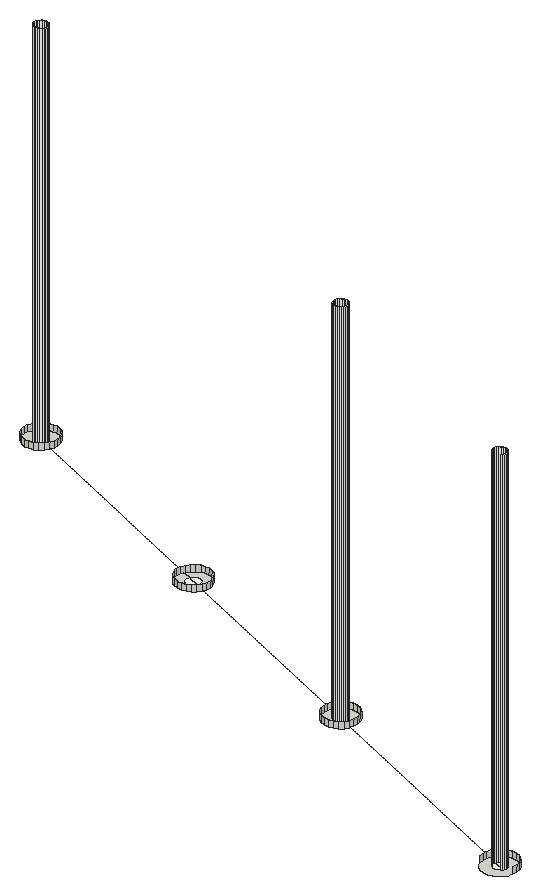
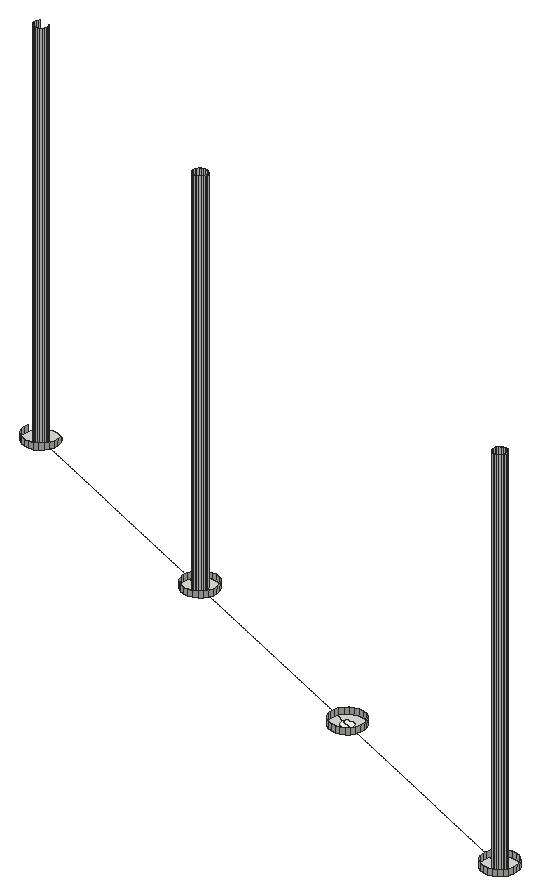
# SketchUp Ruby script. Lengths in inches.
U = 1.inch
M = Sketchup.active_model
def pt(a) = Geom::Point3d.new(a.map { |v| v * U })
def face(e, loops, mat)
  f = e.add_face(loops[0].map { |a| pt(a) })
  loops[1..].each { |l| e.add_face(l.map { |a| pt(a) }).erase! }
  f.material = f.back_material = mat if mat
  f
end
# faces: each face lists its corners as indices into pts; further lists are holes
def faces(e, pts, list, mat = nil) = list.each { |f| face(e, (f[0].is_a?(Array) ? f : [f]).map { |l| l.map { |i| pts[i] } }, mat) }
# xy, xz, yz: faces in a plane at the given z, y or x. An outline is a flat list of corners, or four numbers for a rectangle; further outlines are holes
def ring(l) = l.size == 4 ? [[l[0], l[1]], [l[2], l[1]], [l[2], l[3]], [l[0], l[3]]] : l.each_slice(2).to_a
def flat(e, list, mat, &to3) = list.each { |f| face(e, (f[0].is_a?(Array) ? f : [f]).map { |l| ring(l).map { |u, v| to3.(u, v) } }, mat) }
def xy(e, z, list, mat = nil) = flat(e, list, mat) { |x, y| [x, y, z] }
def xz(e, y, list, mat = nil) = flat(e, list, mat) { |x, z| [x, y, z] }
def yz(e, x, list, mat = nil) = flat(e, list, mat) { |y, z| [x, y, z] }
def lines(e, pts, list) = list.each { |a, b| e.add_line(pt(pts[a]), pt(pts[b])) }
# prism: a flat outline (further loops are holes) pulled along v
def prism(e, loops, v, mat = nil)
  f = face(e, loops, mat); d = Geom::Vector3d.new(v.map { |x| x * U })
  f.pushpull(f.normal.samedirection?(d) ? d.length : -d.length)
end
def box(e, o, s, mat = nil) = prism(e, [[o, [o[0] + s[0], o[1], o[2]], [o[0] + s[0], o[1] + s[1], o[2]], [o[0], o[1] + s[1], o[2]]]], [0, 0, s[2]], mat)
def at(x, y, z, deg = 0) = Geom::Transformation.translation(pt([x, y, z])) * Geom::Transformation.rotation(ORIGIN, Z_AXIS, deg.degrees)
def axes(o, x, y, z) = Geom::Transformation.new([*x, 0, *y, 0, *z, 0, *pt(o).to_a, 1])
def part(name) = M.definitions.add(name)
# library, detail: a bought-in or finely detailed component or shape, given as its bounding box
def library(name, o, s) = part(name).tap { |d| box(d.entities, o, s) }
def detail(e, o, s) = box(e.add_group.entities, o, s)
def put(e, d, t, mat = nil) = e.add_instance(d, t).tap { |i| i.material = mat if mat }
def group(e, t, mat = nil) = e.add_group.tap { |g| g.transformation = t; g.material = mat if mat }.entities
root = M.entities
M.materials.add("[Color_000]").color = [255, 255, 255]
xy(root,321.27,[[[916.82,1057.59,916.41,1057.62,916.02,1057.75,915.68,1057.97,915.4,1058.28,915.22,1058.65,915.14,1059.05,915.16,1059.46,915.29,1059.85,915.52,1060.19,915.83,1060.47,916.19,1060.65,916.6,1060.73,917.01,1060.71,917.4,1060.58,917.74,1060.35,918.01,1060.05,918.2,1059.68,918.28,1059.28,918.25,1058.86,918.15,1058.54,918.125,1058.47,917.9,1058.13,917.59,1057.86,917.22,1057.67],[916.75,1058.53,916.91,1058.57,917.0625,1058.64,917.18,1058.75,917.27,1058.89,917.28,1058.91,917.33,1059.04,917.34,1059.21,917.3,1059.37,917.23,1059.52,917.12,1059.64,916.98,1059.73,916.83,1059.78,916.66,1059.79,916.5,1059.76,916.36,1059.68,916.23,1059.58,916.14,1059.4375,916.13,1059.41,916.09,1059.28,916.08,1059.12,916.11,1058.96,916.1875,1058.81,916.3,1058.6875,916.43,1058.6,916.59,1058.54]],[893.19,1067.88,892.78,1067.91,892.39,1068.04,892.05,1068.26,891.78,1068.57,891.59,1068.9375,891.51,1069.34,891.53,1069.75,891.64,1070.08,892.5,1069.7,892.46,1069.57,892.45,1069.41,892.48,1069.25,892.56,1069.1,892.67,1068.98,892.8,1068.89,892.96,1068.84,893.125,1068.83,893.29,1068.86,893.43,1068.93,893.56,1069.04,893.65,1069.18,893.65,1069.2,894.52,1068.83,894.5,1068.77,894.27,1068.42,893.96,1068.15,893.59,1067.97],[[893.19,1067.88,893.59,1067.97,893.96,1068.15,894.27,1068.42,894.5,1068.77,894.52,1068.83,894.625,1069.16,894.65,1069.57,894.57,1069.97,894.38,1070.34,894.11,1070.64,893.77,1070.87,893.38,1071,892.97,1071.02,892.5625,1070.94,892.2,1070.76,891.89,1070.48,891.66,1070.14,891.53,1069.75,891.51,1069.34,891.59,1068.9375,891.78,1068.57,892.05,1068.26,892.39,1068.04,892.78,1067.91],[893.125,1068.83,892.96,1068.84,892.8,1068.89,892.67,1068.98,892.56,1069.1,892.48,1069.25,892.45,1069.41,892.46,1069.57,892.5,1069.7,892.51,1069.73,892.6,1069.87,892.73,1069.98,892.875,1070.05,893.03,1070.08,893.2,1070.07,893.35,1070.02,893.49,1069.93,893.6,1069.81,893.67,1069.66,893.71,1069.5,893.7,1069.33,893.65,1069.2,893.65,1069.18,893.56,1069.04,893.43,1068.93,893.29,1068.86]],[871.35,1077.4,870.9375,1077.42,870.55,1077.55,870.2,1077.78,869.93,1078.08,869.75,1078.45,869.66,1078.85,869.6875,1079.27,869.8,1079.59,870.66,1079.22,870.62,1079.09,870.61,1078.92,870.64,1078.76,870.71,1078.61,870.82,1078.49,870.96,1078.4,871.12,1078.35,871.28,1078.34,871.44,1078.37,871.59,1078.45,871.71,1078.56,871.8,1078.69,871.81,1078.72,872.67,1078.34,872.65,1078.28,872.43,1077.9375,872.12,1077.66,871.75,1077.48],[[871.35,1077.4,870.9375,1077.42,870.55,1077.55,870.2,1077.78,869.93,1078.08,869.75,1078.45,869.66,1078.85,869.6875,1079.27,869.8,1079.59,869.82,1079.66,870.05,1080,870.35,1080.27,870.72,1080.46,871.12,1080.54,871.53,1080.51,871.92,1080.38,872.27,1080.16,872.54,1079.85,872.72,1079.48,872.81,1079.08,872.78,1078.67,872.65,1078.28,872.43,1077.9375,872.12,1077.66,871.75,1077.48],[871.28,1078.34,871.44,1078.37,871.59,1078.45,871.71,1078.56,871.8,1078.69,871.81,1078.72,871.85,1078.85,871.86,1079.01,871.83,1079.17,871.76,1079.32,871.65,1079.44,871.51,1079.53,871.35,1079.59,871.19,1079.6,871.03,1079.5625,870.88,1079.49,870.76,1079.38,870.67,1079.24,870.66,1079.22,870.62,1079.09,870.61,1078.92,870.64,1078.76,870.71,1078.61,870.82,1078.49,870.96,1078.4,871.12,1078.35]],
  [848.68,1087.27,848.27,1087.29,847.88,1087.42,847.54,1087.65,847.27,1087.96,847.08,1088.32,847,1088.73,847.02,1089.14,847.13,1089.47,847.99,1089.09,847.95,1088.96,847.94,1088.79,847.97,1088.63,848.05,1088.49,848.16,1088.36,848.29,1088.27,848.45,1088.22,848.61,1088.21,848.78,1088.24,848.92,1088.32,849.05,1088.43,849.14,1088.5625,849.14,1088.59,850.01,1088.21,849.99,1088.15,849.76,1087.81,849.45,1087.54,849.08,1087.35],[[848.68,1087.27,848.27,1087.29,847.88,1087.42,847.54,1087.65,847.27,1087.96,847.08,1088.32,847,1088.73,847.02,1089.14,847.15,1089.53,847.38,1089.87,847.6875,1090.14,848.05,1090.33,848.46,1090.41,848.87,1090.39,849.26,1090.26,849.6,1090.03,849.875,1089.72,850.06,1089.35,850.14,1088.95,850.12,1088.54,849.99,1088.15,849.76,1087.81,849.45,1087.54,849.08,1087.35],[848.61,1088.21,848.78,1088.24,848.92,1088.32,849.05,1088.43,849.14,1088.5625,849.14,1088.59,849.1875,1088.72,849.2,1088.88,849.16,1089.05,849.09,1089.19,848.98,1089.32,848.84,1089.41,848.6875,1089.46,848.52,1089.47,848.36,1089.43,848.22,1089.36,848.09,1089.25,848,1089.11,847.99,1089.09,847.95,1088.96,847.94,1088.79,847.97,1088.63,848.05,1088.49,848.16,1088.36,848.29,1088.27,848.45,1088.22]]])
xy(root,321.27,[[916.75,1058.53,916.59,1058.54,916.43,1058.6,916.3,1058.6875,916.1875,1058.81,916.11,1058.96,916.08,1059.12,916.09,1059.28,916.13,1059.41,917.28,1058.91,917.27,1058.89,917.18,1058.75,917.0625,1058.64,916.91,1058.57],[917.28,1058.91,916.13,1059.41,916.14,1059.4375,916.23,1059.58,916.36,1059.68,916.5,1059.76,916.66,1059.79,916.83,1059.78,916.98,1059.73,917.12,1059.64,917.23,1059.52,917.3,1059.37,917.34,1059.21,917.33,1059.04],[893.125,1068.83,892.96,1068.84,892.8,1068.89,892.67,1068.98,892.56,1069.1,892.48,1069.25,892.45,1069.41,892.46,1069.57,892.5,1069.7,893.65,1069.2,893.65,1069.18,893.56,1069.04,893.43,1068.93,893.29,1068.86],[893.65,1069.2,892.5,1069.7,892.51,1069.73,892.6,1069.87,892.73,1069.98,892.875,1070.05,893.03,1070.08,893.2,1070.07,893.35,1070.02,893.49,1069.93,893.6,1069.81,893.67,1069.66,893.71,1069.5,893.7,1069.33],[871.28,1078.34,871.12,1078.35,870.96,1078.4,870.82,1078.49,870.71,1078.61,870.64,1078.76,870.61,1078.92,870.62,1079.09,870.66,1079.22,871.81,1078.72,871.8,1078.69,871.71,1078.56,871.59,1078.45,871.44,1078.37],
  [871.81,1078.72,870.66,1079.22,870.67,1079.24,870.76,1079.38,870.88,1079.49,871.03,1079.5625,871.19,1079.6,871.35,1079.59,871.51,1079.53,871.65,1079.44,871.76,1079.32,871.83,1079.17,871.86,1079.01,871.85,1078.85],[848.61,1088.21,848.45,1088.22,848.29,1088.27,848.16,1088.36,848.05,1088.49,847.97,1088.63,847.94,1088.79,847.95,1088.96,847.99,1089.09,849.14,1088.59,849.14,1088.5625,849.05,1088.43,848.92,1088.32,848.78,1088.24],[849.14,1088.59,847.99,1089.09,848,1089.11,848.09,1089.25,848.22,1089.36,848.36,1089.43,848.52,1089.47,848.6875,1089.46,848.84,1089.41,848.98,1089.32,849.09,1089.19,849.16,1089.05,849.2,1088.88,849.1875,1088.72]],"[Color_000]")
p = [[915.14,1059.05,321.27],[915.22,1058.65,321.27],[915.22,1058.65,321.86],[915.14,1059.05,321.86],[916.11,1058.96,321.27],[916.1875,1058.81,321.27],
  [916.1875,1058.81,357.27],[916.11,1058.96,357.27],[917.18,1058.75,321.27],[917.27,1058.89,321.27],[917.27,1058.89,357.27],[917.18,1058.75,357.27],
  [917.28,1058.91,321.27],[917.33,1059.04,321.27],[917.33,1059.04,357.27],[918.25,1058.86,321.27],[918.28,1059.28,321.27],[918.28,1059.28,321.86],
  [918.25,1058.86,321.86],[916.08,1059.12,321.27],[916.08,1059.12,357.27],[917.34,1059.21,321.27],[917.34,1059.21,357.27],[915.16,1059.46,321.27],
  [915.16,1059.46,321.86],[916.09,1059.28,321.27],[916.09,1059.28,357.27],[917.3,1059.37,321.27],[917.3,1059.37,357.27],[916.14,1059.4375,321.27],
  [916.13,1059.41,321.27],[916.14,1059.4375,357.27],[918.2,1059.68,321.27],[918.2,1059.68,321.86],[916.23,1059.58,321.27],[916.23,1059.58,357.27],
  [917.23,1059.52,321.27],[917.23,1059.52,357.27],[915.29,1059.85,321.27],[915.27,1059.79,321.27],[915.29,1059.85,321.86],[917.12,1059.64,321.27],
  [917.12,1059.64,357.27],[916.36,1059.68,321.27],[916.36,1059.68,357.27],[916.98,1059.73,321.27],[916.98,1059.73,357.27],[916.5,1059.76,321.27],
  [916.5,1059.76,357.27],[916.83,1059.78,321.27],[916.83,1059.78,357.27],[918.01,1060.05,321.27],[918.01,1060.05,321.86],[916.66,1059.79,321.27],
  [916.66,1059.79,357.27],[915.52,1060.19,321.27],[915.52,1060.19,321.86],[917.74,1060.35,321.27],[917.74,1060.35,321.86],[915.83,1060.47,321.27],
  [915.83,1060.47,321.86],[917.4,1060.58,321.27],[917.4,1060.58,321.86],[916.19,1060.65,321.27],[916.19,1060.65,321.86],[917.01,1060.71,321.27],
  [917.01,1060.71,321.86],[916.6,1060.73,321.27],[916.6,1060.73,321.86],[892.39,1068.04,321.27],[892.78,1067.91,321.27],[892.78,1067.91,321.86],
  [892.39,1068.04,321.86],[893.19,1067.88,321.27],[893.19,1067.88,321.86],[893.59,1067.97,321.27],[893.59,1067.97,321.86],[892.05,1068.26,321.27],
  [892.05,1068.26,321.86],[893.96,1068.15,321.27],[893.96,1068.15,321.86],[894.27,1068.42,321.27],[894.27,1068.42,321.86],[891.78,1068.57,321.27],
  [891.78,1068.57,321.86],[894.5,1068.77,321.27],[894.5,1068.77,321.86],[891.59,1068.9375,321.27],[891.59,1068.9375,321.86],[892.8,1068.89,321.27],
  [892.96,1068.84,321.27],[892.96,1068.84,357.27],[892.8,1068.89,357.27],[893.125,1068.83,321.27],[893.125,1068.83,357.27],[893.29,1068.86,321.27],
  [893.29,1068.86,357.27],[894.52,1068.83,321.27],[894.625,1069.16,321.27],[894.625,1069.16,321.86],[891.51,1069.34,321.27],[891.51,1069.34,321.86],
  [892.67,1068.98,321.27],[892.67,1068.98,357.27],[893.43,1068.93,321.27],[893.43,1068.93,357.27],[893.56,1069.04,321.27],[893.56,1069.04,357.27],
  [892.56,1069.1,321.27],[892.56,1069.1,357.27],[893.65,1069.18,321.27],[893.65,1069.18,357.27],[892.48,1069.25,321.27],[892.48,1069.25,357.27],
  [892.45,1069.41,321.27],[892.45,1069.41,357.27],[893.65,1069.2,321.27],[893.7,1069.33,321.27],[893.7,1069.33,357.27],[894.65,1069.57,321.27],
  [894.65,1069.57,321.86],[891.53,1069.75,321.27],[891.53,1069.75,321.86],[893.71,1069.5,321.27],[893.71,1069.5,357.27],[892.46,1069.57,321.27],
  [892.46,1069.57,357.27],[893.67,1069.66,321.27],[893.67,1069.66,357.27],[892.51,1069.73,321.27],[892.5,1069.7,321.27],[892.51,1069.73,357.27],
  [894.57,1069.97,321.27],[894.57,1069.97,321.86],[892.6,1069.87,321.27],[892.6,1069.87,357.27],[893.6,1069.81,321.27],[893.6,1069.81,357.27],
  [891.66,1070.14,321.27],[891.64,1070.08,321.27],[891.66,1070.14,321.86],[893.49,1069.93,321.27],[893.49,1069.93,357.27],[892.73,1069.98,321.27],
  [892.73,1069.98,357.27],[893.35,1070.02,321.27],[893.35,1070.02,357.27],[892.875,1070.05,321.27],[892.875,1070.05,357.27],[893.03,1070.08,321.27],
  [893.03,1070.08,357.27],[893.2,1070.07,321.27],[893.2,1070.07,357.27],[894.38,1070.34,321.27],[894.38,1070.34,321.86],[891.89,1070.48,321.27],
  [891.89,1070.48,321.86],[894.11,1070.64,321.27],[894.11,1070.64,321.86],[892.2,1070.76,321.27],[892.2,1070.76,321.86],[893.77,1070.87,321.27],
  [893.77,1070.87,321.86],[892.5625,1070.94,321.27],[892.5625,1070.94,321.86],[892.97,1071.02,321.27],[892.97,1071.02,321.86],[893.38,1071,321.27],
  [893.38,1071,321.86],[870.55,1077.55,321.27],[870.9375,1077.42,321.27],[870.9375,1077.42,321.86],[870.55,1077.55,321.86],[871.35,1077.4,321.27],
  [871.35,1077.4,321.86],[871.75,1077.48,321.27],[871.75,1077.48,321.86],[872.12,1077.66,321.27],[872.12,1077.66,321.86],[870.2,1077.78,321.27],
  [870.2,1077.78,321.86],[872.43,1077.9375,321.27],[872.43,1077.9375,321.86],[869.93,1078.08,321.27],[869.93,1078.08,321.86],[872.65,1078.28,321.27],
  [872.65,1078.28,321.86],[869.75,1078.45,321.27],[869.75,1078.45,321.86],[872.67,1078.34,321.27],[872.78,1078.67,321.27],[872.78,1078.67,321.86],
  [869.66,1078.85,321.27],[869.66,1078.85,321.86],[872.81,1079.08,321.27],[872.81,1079.08,321.86],[869.6875,1079.27,321.27],[869.6875,1079.27,321.86],
  [872.72,1079.48,321.27],[872.72,1079.48,321.86],[869.82,1079.66,321.27],[869.8,1079.59,321.27],[869.82,1079.66,321.86],[872.54,1079.85,321.27],
  [872.54,1079.85,321.86],[870.05,1080,321.27],[870.05,1080,321.86],[872.27,1080.16,321.27],[872.27,1080.16,321.86],[870.35,1080.27,321.27],
  [870.35,1080.27,321.86],[871.92,1080.38,321.27],[871.92,1080.38,321.86],[870.72,1080.46,321.27],[870.72,1080.46,321.86],[871.53,1080.51,321.27],
  [871.53,1080.51,321.86],[871.12,1080.54,321.27],[871.12,1080.54,321.86],[847.88,1087.42,321.27],[848.27,1087.29,321.27],[848.27,1087.29,321.86],
  [847.88,1087.42,321.86],[848.68,1087.27,321.27],[848.68,1087.27,321.86],[849.08,1087.35,321.27],[849.08,1087.35,321.86],[847.54,1087.65,321.27],
  [847.54,1087.65,321.86],[849.45,1087.54,321.27],[849.45,1087.54,321.86],[849.76,1087.81,321.27],[849.76,1087.81,321.86],[847.27,1087.96,321.27],
  [847.27,1087.96,321.86],[849.99,1088.15,321.27],[849.99,1088.15,321.86],[847.08,1088.32,321.27],[847.08,1088.32,321.86],[848.29,1088.27,321.27],
  [848.45,1088.22,321.27],[848.45,1088.22,357.27],[848.29,1088.27,357.27],[848.61,1088.21,321.27],[848.61,1088.21,357.27],[848.78,1088.24,321.27],
  [848.78,1088.24,357.27],[848.92,1088.32,321.27],[848.92,1088.32,357.27],[850.01,1088.21,321.27],[850.12,1088.54,321.27],[850.12,1088.54,321.86],
  [847,1088.73,321.27],[847,1088.73,321.86],[848.16,1088.36,321.27],[848.16,1088.36,357.27],[849.05,1088.43,321.27],[849.05,1088.43,357.27],
  [848.05,1088.49,321.27],[848.05,1088.49,357.27],[849.14,1088.5625,321.27],[849.14,1088.5625,357.27],[847.97,1088.63,321.27],[847.97,1088.63,357.27],
  [850.14,1088.95,321.27],[850.14,1088.95,321.86],[847.94,1088.79,321.27],[847.94,1088.79,357.27],[849.14,1088.59,321.27],[849.1875,1088.72,321.27],
  [849.1875,1088.72,357.27],[847.02,1089.14,321.27],[847.02,1089.14,321.86],[849.2,1088.88,321.27],[849.2,1088.88,357.27],[847.95,1088.96,321.27],
  [847.95,1088.96,357.27],[849.16,1089.05,321.27],[849.16,1089.05,357.27],[848,1089.11,321.27],[847.99,1089.09,321.27],[848,1089.11,357.27],
  [849.09,1089.19,321.27],[849.09,1089.19,357.27],[850.06,1089.35,321.27],[850.06,1089.35,321.86],[847.15,1089.53,321.27],[847.13,1089.47,321.27],
  [847.15,1089.53,321.86],[848.09,1089.25,321.27],[848.09,1089.25,357.27],[848.98,1089.32,321.27],[848.98,1089.32,357.27],[848.22,1089.36,321.27],
  [848.22,1089.36,357.27],[848.84,1089.41,321.27],[848.84,1089.41,357.27],[848.36,1089.43,321.27],[848.36,1089.43,357.27],[848.52,1089.47,321.27],
  [848.52,1089.47,357.27],[848.6875,1089.46,321.27],[848.6875,1089.46,357.27],[849.875,1089.72,321.27],[849.875,1089.72,321.86],[847.38,1089.87,321.27],
  [847.38,1089.87,321.86],[849.6,1090.03,321.27],[849.6,1090.03,321.86],[847.6875,1090.14,321.27],[847.6875,1090.14,321.86],[849.26,1090.26,321.27],
  [849.26,1090.26,321.86],[848.05,1090.33,321.27],[848.05,1090.33,321.86],[848.46,1090.41,321.27],[848.46,1090.41,321.86],[848.87,1090.39,321.27],
  [848.87,1090.39,321.86]]
faces(root,p,[[0,1,2,3],[15,16,17,18],[23,0,3,24],[16,32,33,17],[38,39,23,24,40],[32,51,52,33],[55,38,40,56],[51,57,58,52],
  [59,55,56,60],[57,61,62,58],[63,59,60,64],[61,65,66,62],[67,63,64,68],[65,67,68,66],[69,70,71,72],[70,73,74,71],
  [73,75,76,74],[77,69,72,78],[75,79,80,76],[79,81,82,80],[83,77,78,84],[81,85,86,82],[87,83,84,88],[85,97,98,99,86],
  [100,87,88,101],[98,119,120,99],[121,100,101,122],[119,132,133,120],[138,139,121,122,140],[132,153,154,133],[155,138,140,156],[153,157,158,154],
  [159,155,156,160],[157,161,162,158],[163,159,160,164],[165,163,164,166],[161,167,168,162],[167,165,166,168],[169,170,171,172],[170,173,174,171],
  [173,175,176,174],[175,177,178,176],[179,169,172,180],[177,181,182,178],[183,179,180,184],[181,185,186,182],[187,183,184,188],[185,189,190,191,186],
  [192,187,188,193],[190,194,195,191],[196,192,193,197],[194,198,199,195],[200,201,196,197,202],[198,203,204,199],[205,200,202,206],[203,207,208,204],
  [209,205,206,210],[207,211,212,208],[213,209,210,214],[211,215,216,212],[217,213,214,218],[215,217,218,216],[219,220,221,222],[220,223,224,221],
  [223,225,226,224],[227,219,222,228],[225,229,230,226],[229,231,232,230],[233,227,228,234],[231,235,236,232],[237,233,234,238],[235,249,250,251,236],
  [252,237,238,253],[250,264,265,251],[271,252,253,272],[264,284,285,265],[286,287,271,272,288],[284,303,304,285],[305,286,288,306],[303,307,308,304],
  [309,305,306,310],[307,311,312,308],[313,309,310,314],[315,313,314,316],[311,317,318,312],[317,315,316,318]])
faces(root,p,[[4,5,6,7],[8,9,10,11],[9,12,13,14,10],[19,4,7,20],[13,21,22,14],[25,19,20,26],[21,27,28,22],[29,30,25,26,31],
  [34,29,31,35],[27,36,37,28],[36,41,42,37],[43,34,35,44],[41,45,46,42],[47,43,44,48],[45,49,50,46],[53,47,48,54],
  [49,53,54,50],[89,90,91,92],[90,93,94,91],[93,95,96,94],[102,89,92,103],[95,104,105,96],[104,106,107,105],[108,102,103,109],
  [106,110,111,107],[112,108,109,113],[114,112,113,115],[110,116,117,118,111],[117,123,124,118],[125,114,115,126],[123,127,128,124],[129,130,125,126,131],
  [134,129,131,135],[127,136,137,128],[136,141,142,137],[143,134,135,144],[141,145,146,142],[147,143,144,148],[149,147,148,150],[145,151,152,146],
  [151,149,150,152],[239,240,241,242],[240,243,244,241],[243,245,246,244],[245,247,248,246],[254,239,242,255],[247,256,257,248],[258,254,255,259],
  [256,260,261,257],[262,258,259,263],[266,262,263,267],[260,268,269,270,261],[269,273,274,270],[275,266,267,276],[273,277,278,274],[279,280,275,276,281],
  [277,282,283,278],[289,279,281,290],[282,291,292,283],[293,289,290,294],[291,295,296,292],[297,293,294,298],[299,297,298,300],[295,301,302,296],
  [301,299,300,302]],"[Color_000]")
lines(root,p,[[39,97],[139,189],[201,249]])
